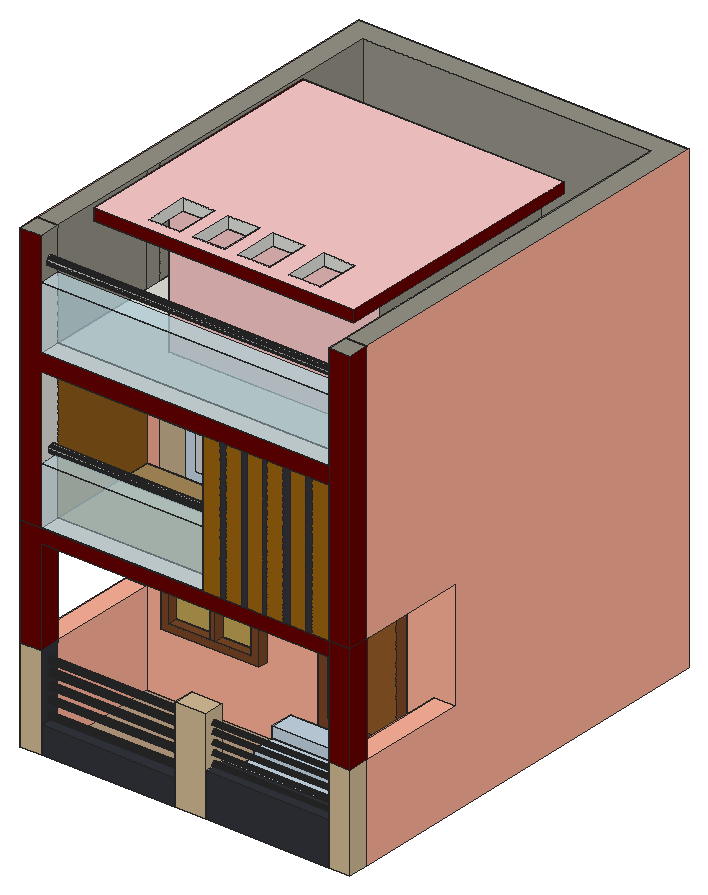
# SketchUp Ruby script. Lengths in inches.
U = 1.inch
M = Sketchup.active_model
def pt(a) = Geom::Point3d.new(a.map { |v| v * U })
def face(e, loops, mat)
  f = e.add_face(loops[0].map { |a| pt(a) })
  loops[1..].each { |l| e.add_face(l.map { |a| pt(a) }).erase! }
  f.material = f.back_material = mat if mat
  f
end
# faces: each face lists its corners as indices into pts; further lists are holes
def faces(e, pts, list, mat = nil) = list.each { |f| face(e, (f[0].is_a?(Array) ? f : [f]).map { |l| l.map { |i| pts[i] } }, mat) }
# xy, xz, yz: faces in a plane at the given z, y or x. An outline is a flat list of corners, or four numbers for a rectangle; further outlines are holes
def ring(l) = l.size == 4 ? [[l[0], l[1]], [l[2], l[1]], [l[2], l[3]], [l[0], l[3]]] : l.each_slice(2).to_a
def flat(e, list, mat, &to3) = list.each { |f| face(e, (f[0].is_a?(Array) ? f : [f]).map { |l| ring(l).map { |u, v| to3.(u, v) } }, mat) }
def xy(e, z, list, mat = nil) = flat(e, list, mat) { |x, y| [x, y, z] }
def xz(e, y, list, mat = nil) = flat(e, list, mat) { |x, z| [x, y, z] }
def yz(e, x, list, mat = nil) = flat(e, list, mat) { |y, z| [x, y, z] }
def lines(e, pts, list) = list.each { |a, b| e.add_line(pt(pts[a]), pt(pts[b])) }
# prism: a flat outline (further loops are holes) pulled along v
def prism(e, loops, v, mat = nil)
  f = face(e, loops, mat); d = Geom::Vector3d.new(v.map { |x| x * U })
  f.pushpull(f.normal.samedirection?(d) ? d.length : -d.length)
end
def box(e, o, s, mat = nil) = prism(e, [[o, [o[0] + s[0], o[1], o[2]], [o[0] + s[0], o[1] + s[1], o[2]], [o[0], o[1] + s[1], o[2]]]], [0, 0, s[2]], mat)
def at(x, y, z, deg = 0) = Geom::Transformation.translation(pt([x, y, z])) * Geom::Transformation.rotation(ORIGIN, Z_AXIS, deg.degrees)
def axes(o, x, y, z) = Geom::Transformation.new([*x, 0, *y, 0, *z, 0, *pt(o).to_a, 1])
def part(name) = M.definitions.add(name)
# library, detail: a bought-in or finely detailed component or shape, given as its bounding box
def library(name, o, s) = part(name).tap { |d| box(d.entities, o, s) }
def detail(e, o, s) = box(e.add_group.entities, o, s)
def put(e, d, t, mat = nil) = e.add_instance(d, t).tap { |i| i.material = mat if mat }
def group(e, t, mat = nil) = e.add_group.tap { |g| g.transformation = t; g.material = mat if mat }.entities
root = M.entities
M.materials.add("[Aluminum]").color = [179, 179, 179]
M.materials.add("[Blinds Cloth Horizontal]").color = [192, 163, 85]
M.materials.add("[Blinds Vertical Pattern]").color = [212, 212, 214]
M.materials.add("[Blinds Weave]").color = [141, 91, 25]
M.materials.add("[Blinds Wood Light]").color = [155, 100, 14]
M.materials.add("[Carpet Loop Pattern]").color = [166, 138, 89]
M.materials.add("[Carpet Pattern Leaf Squares Tan]").color = [181, 154, 125]
M.materials.add("[Color A01]").color = [255, 204, 204]
M.materials.add("[Color A08]").color = [102, 0, 0]
M.materials.add("[Color B02]").color = [255, 178, 153]
M.materials.add("[Color M08]").color = [30, 30, 30]
M.materials.add("[Formica Beige]").color = [211, 187, 149]
M.materials.add("[Formica Graystone]").color = [149, 146, 135]
M.materials.add("[Formica Laminate Dark]").color = [50, 53, 60]
M.materials.add("[Terrazzo Light Blue]").color = [196, 214, 227]
M.materials.add("[Translucent Glass Safety]").color = [204, 235, 244]
M.materials["[Translucent Glass Safety]"].alpha = 0.5
M.materials.add("[Wood Bamboo]").color = [177, 105, 43]
M.materials.add("[Wood Floor Light]").color = [204, 176, 127]
M.materials.add("[Wood Floor Parquet]").color = [145, 89, 39]
M.materials.add("[Wood Veneer 01]").color = [120, 70, 37]
xy(root,0,[[0,0,4.9375,4.9375],[4.9375,0,36.06,4.9375],[36.06,0,43.13,4.9375],[43.13,0,71.8125,4.9375],[71.8125,0,76.75,4.9375],
  [0,4.9375,4.9375,30.76],[71.8125,4.9375,76.75,30.76],[38.375,14.73,71.8125,20.02],[38.375,20.02,71.8125,25.31],[38.375,25.31,71.8125,30.76],
  [[0,30.76,76.75,98.62],[4.9375,34.47,71.8125,93.68]],[4.9375,34.47,71.8125,93.68]])
xy(root,0,[[4.9375,4.9375,71.8125,4.9375,71.8125,14.73,38.375,14.73,38.375,30.76,4.9375,30.76]],"[Carpet Pattern Leaf Squares Tan]")
xy(root,2.625,[[38.375,14.73,71.8125,20.02]],"[Terrazzo Light Blue]")
xy(root,4.125,[[38.375,20.02,71.8125,25.31]],"[Terrazzo Light Blue]")
xy(root,6.25,[[4.9375,0,36.06,4.9375]],"[Formica Laminate Dark]")
xy(root,6.61,[[44.6,30.76,65.48,34.47]])
xy(root,6.61,[[38.375,25.31,71.8125,30.76]],"[Terrazzo Light Blue]")
xy(root,10,[[43.13,0,71.8125,4.9375]],"[Formica Laminate Dark]")
xy(root,15.55,[[9.99,28.51,32.74,30.76]])
xy(root,17.3,[[21.37,28.51,22.64,30.76]])
xy(root,17.3,[[11.74,28.51,21.37,30.76],[22.64,28.51,31,30.76]],"[Wood Veneer 01]")
xy(root,21.74,[[0,0,4.9375,4.9375]])
xy(root,21.74,[[0,4.9375,4.9375,30.76]],"[Color B02]")
xy(root,21.97,[[71.8125,0,76.75,4.9375]])
xy(root,21.97,[[71.8125,4.9375,76.75,30.76]],"[Color B02]")
xy(root,21.97,[[36.06,0,43.13,4.9375]],"[Formica Beige]")
xy(root,37.87,[[11.74,28.51,21.37,30.76],[21.37,28.51,22.64,30.76],[22.64,28.51,31,30.76]])
xy(root,39.61,[[9.99,28.51,32.74,30.76]],"[Wood Veneer 01]")
xy(root,43.9375,[[4.9375,0,71.8125,4.9375],[4.9375,4.9375,71.8125,30.76]],"[Color A01]")
xy(root,44.67,[[44.6,30.76,65.48,34.47]])
xy(root,47.375,[[0,0,4.9375,4.9375],[4.9375,0,42.62,4.9375],[42.62,0,71.8125,4.9375],[71.8125,0,76.75,4.9375]])
xy(root,47.375,[[4.9375,4.9375,71.8125,30.76]],"[Carpet Loop Pattern]")
xy(root,47.375,[[0,4.9375,4.9375,30.76],[71.8125,4.9375,76.75,30.76]],"[Color A01]")
xy(root,60.75,[[4.9375,0,42.62,4.9375]],"[Translucent Glass Safety]")
xy(root,79.89,[[4.9375,0,42.62,4.9375]])
xy(root,83.8125,[[4.9375,0,71.8125,4.9375],[4.9375,4.9375,71.8125,4.9375,71.8125,15.02,22.6875,15.02,22.6875,61.77,71.8125,61.77,71.8125,93.68,4.9375,93.68],[22.6875,15.02,71.8125,61.77]])
xy(root,98.5625,[[4.9375,0,71.8125,4.9375]],"[Translucent Glass Safety]")
xy(root,108.3125,[[0,0,4.9375,4.9375],[71.8125,0,76.75,4.9375],[0,4.9375,4.9375,4.9375,4.9375,93.68,71.8125,93.68,71.8125,4.9375,76.75,4.9375,76.75,98.62,0,98.62]],"[Formica Graystone]")
xy(root,115.22,[[35.52,1.27,35.28,1.3,35.05,1.39,34.86,1.54,34.71,1.73,34.61,1.96,34.58,2.2,34.61,2.45,34.71,2.67,34.86,2.87,35.05,3.01,35.28,3.11,35.52,3.14,35.76,3.11,35.99,3.01,36.18,2.87,36.33,2.67,36.42,2.45,36.46,2.2,36.42,1.96,36.33,1.73,36.18,1.54,35.99,1.39,35.76,1.3],[45.96,1.27,45.71,1.3,45.49,1.39,45.29,1.54,45.14,1.73,45.05,1.96,45.02,2.2,45.05,2.45,45.14,2.67,45.29,2.87,45.49,3.01,45.71,3.11,45.96,3.14,46.2,3.11,46.43,3.01,46.62,2.87,46.77,2.67,46.86,2.45,46.89,2.2,46.86,1.96,46.77,1.73,46.62,1.54,46.43,1.39,46.2,1.3],[56.89,1.27,56.65,1.3,56.43,1.39,56.23,1.54,56.08,1.73,55.99,1.96,55.96,2.2,55.99,2.45,56.08,2.67,56.23,2.87,56.43,3.01,56.65,3.11,56.89,3.14,57.14,3.11,57.36,3.01,57.56,2.87,57.71,2.67,57.8,2.45,57.83,2.2,57.8,1.96,57.71,1.73,57.56,1.54,57.36,1.39,57.14,1.3],[72.48,2.38,72.24,2.41,72.01,2.5,71.82,2.65,71.67,2.85,71.57,3.07,71.54,3.32,71.57,3.56,71.67,3.78,71.82,3.98,72.01,4.13,72.24,4.22,72.48,4.25,72.72,4.22,72.95,4.13,73.14,3.98,73.29,3.78,73.38,3.56,73.42,3.32,73.38,3.07,73.29,2.85,73.14,2.65,72.95,2.5,72.72,2.41],[20.14,3.18,19.89,3.21,19.67,3.31,19.47,3.46,19.33,3.65,19.23,3.875,19.2,4.12,19.23,4.36,19.33,4.59,19.47,4.78,19.67,4.93,19.89,5.02,20.14,5.06,20.38,5.02,20.61,4.93,20.8,4.78,20.95,4.59,21.04,4.36,21.08,4.12,21.04,3.875,20.95,3.65,20.8,3.46,20.61,3.31,20.38,3.21]])
xy(root,115.22,[[[16.5,0.77,16.5,61.77,22.6875,61.77,22.6875,15.02,71.8125,15.02,71.8125,61.77,77.125,61.77,77.125,0.77],[26.97,3.62,34.28,13.74],[37.41,3.62,44.72,13.74],[47.91,3.62,55.22,13.74],[59.66,3.62,66.97,13.74],[20.14,3.18,20.38,3.21,20.61,3.31,20.8,3.46,20.95,3.65,21.04,3.875,21.08,4.12,21.04,4.36,20.95,4.59,20.8,4.78,20.61,4.93,20.38,5.02,20.14,5.06,19.89,5.02,19.67,4.93,19.47,4.78,19.33,4.59,19.23,4.36,19.2,4.12,19.23,3.875,19.33,3.65,19.47,3.46,19.67,3.31,19.89,3.21],[35.52,1.27,35.76,1.3,35.99,1.39,36.18,1.54,36.33,1.73,36.42,1.96,36.46,2.2,36.42,2.45,36.33,2.67,36.18,2.87,35.99,3.01,35.76,3.11,35.52,3.14,35.28,3.11,35.05,3.01,34.86,2.87,34.71,2.67,34.61,2.45,34.58,2.2,34.61,1.96,34.71,1.73,34.86,1.54,35.05,1.39,35.28,1.3],[45.96,1.27,46.2,1.3,46.43,1.39,46.62,1.54,46.77,1.73,46.86,1.96,46.89,2.2,46.86,2.45,46.77,2.67,46.62,2.87,46.43,3.01,46.2,3.11,45.96,3.14,45.71,3.11,45.49,3.01,45.29,2.87,45.14,2.67,45.05,2.45,45.02,2.2,45.05,1.96,45.14,1.73,45.29,1.54,45.49,1.39,45.71,1.3],[56.89,1.27,57.14,1.3,57.36,1.39,57.56,1.54,57.71,1.73,57.8,1.96,57.83,2.2,57.8,2.45,57.71,2.67,57.56,2.87,57.36,3.01,57.14,3.11,56.89,3.14,56.65,3.11,56.43,3.01,56.23,2.87,56.08,2.67,55.99,2.45,55.96,2.2,55.99,1.96,56.08,1.73,56.23,1.54,56.43,1.39,56.65,1.3],[72.48,2.38,72.72,2.41,72.95,2.5,73.14,2.65,73.29,2.85,73.38,3.07,73.42,3.32,73.38,3.56,73.29,3.78,73.14,3.98,72.95,4.13,72.72,4.22,72.48,4.25,72.24,4.22,72.01,4.13,71.82,3.98,71.67,3.78,71.57,3.56,71.54,3.32,71.57,3.07,71.67,2.85,71.82,2.65,72.01,2.5,72.24,2.41]]],"[Color A08]")
xy(root,117.875,[[[16.5,0.77,77.125,61.77],[26.97,3.62,34.28,13.74],[37.41,3.62,44.72,13.74],[47.91,3.62,55.22,13.74],[59.66,3.62,66.97,13.74]]],"[Color A01]")
xz(root,0,[[42.62,47.375,46.39,79.89],[47.81,47.375,51.58,79.89],[52.68,47.375,56.45,79.89],[57.49,47.375,61.27,79.89],[62.77,47.375,66.54,79.89],
  [68.04,47.375,71.8125,79.89]],"[Blinds Wood Light]")
xz(root,0,[[0,21.74,4.9375,21.74,4.9375,43.9375,71.8125,43.9375,71.8125,47.375,0,47.375],[71.8125,21.97,76.75,47.375],[0,47.375,4.9375,47.375,4.9375,79.89,71.8125,79.89,71.8125,83.8125,4.9375,83.8125,4.9375,108.3125,0,108.3125],[71.8125,47.375,76.75,108.3125]],"[Color A08]")
xz(root,0,[[0,0,4.9375,21.74],[36.06,0,43.13,21.97],[71.8125,0,76.75,21.97]],"[Formica Beige]")
xz(root,0,[[4.9375,0,36.06,6.25],[43.13,0,71.8125,10],[46.39,47.375,47.81,79.89],[51.58,47.375,52.68,79.89],[56.45,47.375,57.49,79.89],
  [61.27,47.375,62.77,79.89],[66.54,47.375,68.04,79.89]],"[Formica Laminate Dark]")
xz(root,0,[[4.9375,47.375,42.62,60.75],[4.9375,83.8125,71.8125,98.5625]],"[Translucent Glass Safety]")
xz(root,0.77,[[16.5,115.22,77.125,117.875]],"[Color A08]")
xz(root,3.62,[[26.97,115.22,34.28,117.875],[37.41,115.22,44.72,117.875],[47.91,115.22,55.22,117.875],[59.66,115.22,66.97,117.875]])
xz(root,4.9375,[[0,0,4.9375,21.74],[71.8125,0,76.75,21.97],[4.9375,43.9375,71.8125,47.375],[0,47.375,4.9375,83.8125],[42.62,47.375,71.8125,79.89],
  [71.8125,47.375,76.75,83.8125],[4.9375,79.89,71.8125,83.8125],[0,83.8125,4.9375,108.3125],[71.8125,83.8125,76.75,108.3125]])
xz(root,4.9375,[[0,21.74,4.9375,47.375],[71.8125,21.97,76.75,47.375]],"[Color A08]")
xz(root,4.9375,[[36.06,0,43.13,21.97]],"[Formica Beige]")
xz(root,4.9375,[[4.9375,0,36.06,6.25],[43.13,0,71.8125,10]],"[Formica Laminate Dark]")
xz(root,4.9375,[[4.9375,47.375,42.62,60.75],[4.9375,83.8125,71.8125,98.5625]],"[Translucent Glass Safety]")
xz(root,13.74,[[26.97,115.22,34.28,117.875],[37.41,115.22,44.72,117.875],[47.91,115.22,55.22,117.875],[59.66,115.22,66.97,117.875]])
xz(root,14.73,[[38.375,0,71.8125,2.625]],"[Terrazzo Light Blue]")
xz(root,15.02,[[22.6875,83.8125,71.8125,115.22]],"[Color A01]")
xz(root,20.02,[[38.375,0,71.8125,2.625]])
xz(root,20.02,[[38.375,2.625,71.8125,4.125]],"[Terrazzo Light Blue]")
xz(root,25.31,[[38.375,0,71.8125,4.125]])
xz(root,25.31,[[38.375,4.125,71.8125,6.61]],"[Terrazzo Light Blue]")
xz(root,28.51,[[[9.99,15.55,32.74,39.61],[11.74,17.3,31,37.87]],[21.37,17.3,22.64,37.87]],"[Wood Veneer 01]")
xz(root,30.76,[[0,0,4.9375,21.74],[38.375,0,71.8125,6.61],[[9.99,15.55,32.74,39.61],[11.74,17.3,31,37.87]],[21.37,17.3,22.64,37.87],[4.9375,43.9375,13.96,47.375],
  [13.96,43.9375,38.375,47.375],[38.375,43.9375,38.375,47.375,71.8125,47.375,71.8125,43.9375,65.48,43.9375,65.48,44.67,44.6,44.67,44.6,43.9375],[24.93,66.4,25.43,70.52],[26.99,66.4,27.49,70.52]])
xz(root,30.76,[[11.74,17.3,21.37,37.87],[22.64,17.3,31,37.87]],"[Blinds Cloth Horizontal]")
xz(root,30.76,[[16.02,49.43,24.11,78],[28.23,49.43,36.32,78]],"[Blinds Vertical Pattern]")
xz(root,30.76,[[[4.9375,0,38.375,0,38.375,6.61,44.6,6.61,44.6,43.9375,4.9375,43.9375,4.9375,47.375,0,47.375,0,21.74,4.9375,21.74],[9.99,15.55,32.74,39.61]],[65.48,6.61,71.8125,6.61,71.8125,21.97,76.75,21.97,76.75,47.375,71.8125,47.375,71.8125,43.9375,65.48,43.9375]],"[Color B02]")
xz(root,30.76,[[[13.96,47.375,26.17,80.06],[16.02,49.43,24.11,78],[24.93,66.4,25.43,70.52]],[[26.17,47.375,38.375,80.06],[28.23,49.43,36.32,78],[26.99,66.4,27.49,70.52]]],"[Terrazzo Light Blue]")
xz(root,30.76,[[48.54,21.62,49.85,31.37]],"[Wood Floor Light]")
xz(root,30.76,[[[47.12,9.13,62.96,42.15],[48.54,21.62,49.85,31.37]]],"[Wood Floor Parquet]")
xz(root,30.76,[[[44.6,6.61,65.48,43.9375],[47.12,9.13,62.96,42.15]],[44.6,43.9375,65.48,44.67]],"[Wood Veneer 01]")
xz(root,61.77,[[22.6875,83.8125,22.6875,115.22,16.5,115.22,16.5,117.875,77.125,117.875,77.125,115.22,71.8125,115.22,71.8125,83.8125]],"[Color A01]")
xz(root,93.68,[[4.9375,0,71.8125,83.8125]],"[Formica Beige]")
xz(root,93.68,[[4.9375,83.8125,71.8125,108.3125]],"[Formica Graystone]")
xz(root,98.62,[[0,0,76.75,108.3125]],"[Color B02]")
yz(root,0,[[0,21.74,4.9375,47.375],[0,47.375,4.9375,108.3125]],"[Color A08]")
yz(root,0,[[0,0,4.9375,21.74],[30.76,0,30.76,47.375,4.9375,47.375,4.9375,108.3125,98.62,108.3125,98.62,0],[4.9375,0,30.76,21.74]],"[Color B02]")
yz(root,4.9375,[[0,0,4.9375,6.25],[2.57,6.51,2.39,6.54,2.22,6.61,2.08,6.72,1.97,6.86,1.9,7.02,1.88,7.2,1.9,7.38,1.97,7.55,2.08,7.6875,2.22,7.8,2.39,7.87,2.57,7.89,2.74,7.87,2.91,7.8,3.05,7.6875,3.16,7.55,3.23,7.38,3.25,7.2,3.23,7.02,3.16,6.86,3.05,6.72,2.91,6.61,2.74,6.54],[2.57,9.83,2.39,9.85,2.22,9.92,2.08,10.03,1.97,10.17,1.9,10.34,1.88,10.51,1.9,10.69,1.97,10.86,2.08,11,2.22,11.11,2.39,11.18,2.57,11.2,2.74,11.18,2.91,11.11,3.05,11,3.16,10.86,3.23,10.69,3.25,10.51,3.23,10.34,3.16,10.17,3.05,10.03,2.91,9.92,2.74,9.85],[2.57,12.64,2.39,12.66,2.22,12.73,2.08,12.84,1.97,12.98,1.9,13.15,1.88,13.33,1.9,13.51,1.97,13.67,2.08,13.8125,2.22,13.92,2.39,13.99,2.57,14.01,2.74,13.99,2.91,13.92,3.05,13.8125,3.16,13.67,3.23,13.51,3.25,13.33,3.23,13.15,3.16,12.98,3.05,12.84,2.91,12.73,2.74,12.66],[2.57,15.51,2.39,15.54,2.22,15.61,2.08,15.72,1.97,15.86,1.9,16.02,1.88,16.2,1.9,16.38,1.97,16.55,2.08,16.6875,2.22,16.8,2.39,16.87,2.57,16.89,2.74,16.87,2.91,16.8,3.05,16.6875,3.16,16.55,3.23,16.38,3.25,16.2,3.23,16.02,3.16,15.86,3.05,15.72,2.91,15.61,2.74,15.54],
  [2.57,18.08,2.39,18.1,2.22,18.17,2.08,18.28,1.97,18.42,1.9,18.59,1.88,18.76,1.9,18.94,1.97,19.11,2.08,19.25,2.22,19.36,2.39,19.43,2.57,19.45,2.74,19.43,2.91,19.36,3.05,19.25,3.16,19.11,3.23,18.94,3.25,18.76,3.23,18.59,3.16,18.42,3.05,18.28,2.91,18.17,2.74,18.1],[4.9375,43.9375,30.76,47.375],[0,47.375,4.9375,60.75],[[0,60.75,4.9375,79.89],[2.8,61.9,2.56,61.93,2.33,62.02,2.14,62.17,1.99,62.37,1.9,62.59,1.86,62.84,1.9,63.08,1.99,63.3,2.14,63.5,2.33,63.65,2.56,63.74,2.8,63.77,3.04,63.74,3.27,63.65,3.46,63.5,3.61,63.3,3.71,63.08,3.74,62.84,3.71,62.59,3.61,62.37,3.46,62.17,3.27,62.02,3.04,61.93]],[0,83.8125,4.9375,98.5625],
  [2.36,101.3,2.12,101.34,1.89,101.43,1.7,101.58,1.55,101.77,1.45,102,1.42,102.24,1.45,102.48,1.55,102.71,1.7,102.9,1.89,103.05,2.12,103.15,2.36,103.18,2.6,103.15,2.83,103.05,3.02,102.9,3.17,102.71,3.26,102.48,3.3,102.24,3.26,102,3.17,101.77,3.02,101.58,2.83,101.43,2.6,101.34]])
yz(root,4.9375,[[4.9375,47.375,30.76,83.8125]],"[Blinds Weave]")
yz(root,4.9375,[[0,21.74,4.9375,43.9375]],"[Color A08]")
yz(root,4.9375,[[4.9375,0,30.76,21.74]],"[Color B02]")
yz(root,4.9375,[[34.47,0,93.68,83.8125]],"[Formica Beige]")
yz(root,4.9375,[[4.9375,83.8125,30.76,108.3125],[30.76,83.8125,34.47,108.3125],[34.47,83.8125,93.68,108.3125],[[0,98.5625,4.9375,108.3125],[2.36,101.3,2.12,101.34,1.89,101.43,1.7,101.58,1.55,101.77,1.45,102,1.42,102.24,1.45,102.48,1.55,102.71,1.7,102.9,1.89,103.05,2.12,103.15,2.36,103.18,2.6,103.15,2.83,103.05,3.02,102.9,3.17,102.71,3.26,102.48,3.3,102.24,3.26,102,3.17,101.77,3.02,101.58,2.83,101.43,2.6,101.34]]],"[Formica Graystone]")
yz(root,4.9375,[[[0,6.25,4.9375,21.74],[2.57,18.08,2.39,18.1,2.22,18.17,2.08,18.28,1.97,18.42,1.9,18.59,1.88,18.76,1.9,18.94,1.97,19.11,2.08,19.25,2.22,19.36,2.39,19.43,2.57,19.45,2.74,19.43,2.91,19.36,3.05,19.25,3.16,19.11,3.23,18.94,3.25,18.76,3.23,18.59,3.16,18.42,3.05,18.28,2.91,18.17,2.74,18.1],[2.57,15.51,2.39,15.54,2.22,15.61,2.08,15.72,1.97,15.86,1.9,16.02,1.88,16.2,1.9,16.38,1.97,16.55,2.08,16.6875,2.22,16.8,2.39,16.87,2.57,16.89,2.74,16.87,2.91,16.8,3.05,16.6875,3.16,16.55,3.23,16.38,3.25,16.2,3.23,16.02,3.16,15.86,3.05,15.72,2.91,15.61,2.74,15.54],[2.57,12.64,2.39,12.66,2.22,12.73,2.08,12.84,1.97,12.98,1.9,13.15,1.88,13.33,1.9,13.51,1.97,13.67,2.08,13.8125,2.22,13.92,2.39,13.99,2.57,14.01,2.74,13.99,2.91,13.92,3.05,13.8125,3.16,13.67,3.23,13.51,3.25,13.33,3.23,13.15,3.16,12.98,3.05,12.84,2.91,12.73,2.74,12.66],[2.57,9.83,2.39,9.85,2.22,9.92,2.08,10.03,1.97,10.17,1.9,10.34,1.88,10.51,1.9,10.69,1.97,10.86,2.08,11,2.22,11.11,2.39,11.18,2.57,11.2,2.74,11.18,2.91,11.11,3.05,11,3.16,10.86,3.23,10.69,3.25,10.51,3.23,10.34,3.16,10.17,3.05,10.03,2.91,9.92,2.74,9.85],[2.57,6.51,2.39,6.54,2.22,6.61,2.08,6.72,1.97,6.86,1.9,7.02,1.88,7.2,1.9,7.38,1.97,7.55,2.08,7.6875,2.22,7.8,2.39,7.87,2.57,7.89,2.74,7.87,2.91,7.8,3.05,7.6875,3.16,7.55,3.23,7.38,3.25,7.2,3.23,7.02,3.16,6.86,3.05,6.72,2.91,6.61,2.74,6.54]]],"[Formica Laminate Dark]")
yz(root,9.99,[[28.51,15.55,30.76,39.61]],"[Wood Veneer 01]")
yz(root,11.74,[[28.51,17.3,30.76,37.87]],"[Wood Veneer 01]")
yz(root,16.5,[[0.77,115.22,61.77,117.875]],"[Color A08]")
yz(root,21.37,[[28.51,17.3,30.76,37.87]],"[Wood Veneer 01]")
yz(root,22.64,[[28.51,17.3,30.76,37.87]],"[Wood Veneer 01]")
yz(root,22.6875,[[15.02,83.8125,61.77,115.22]],"[Color A01]")
yz(root,26.97,[[3.62,115.22,13.74,117.875]])
yz(root,31,[[28.51,17.3,30.76,37.87]],"[Wood Veneer 01]")
yz(root,32.74,[[28.51,15.55,30.76,39.61]],"[Wood Veneer 01]")
yz(root,34.28,[[3.62,115.22,13.74,117.875]])
yz(root,36.06,[[0,0,4.9375,6.25]])
yz(root,36.06,[[[0,6.25,4.9375,21.97],[2.57,18.08,2.74,18.1,2.91,18.17,3.05,18.28,3.16,18.42,3.23,18.59,3.25,18.76,3.23,18.94,3.16,19.11,3.05,19.25,2.91,19.36,2.74,19.43,2.57,19.45,2.39,19.43,2.22,19.36,2.08,19.25,1.97,19.11,1.9,18.94,1.88,18.76,1.9,18.59,1.97,18.42,2.08,18.28,2.22,18.17,2.39,18.1],[2.57,15.51,2.74,15.54,2.91,15.61,3.05,15.72,3.16,15.86,3.23,16.02,3.25,16.2,3.23,16.38,3.16,16.55,3.05,16.6875,2.91,16.8,2.74,16.87,2.57,16.89,2.39,16.87,2.22,16.8,2.08,16.6875,1.97,16.55,1.9,16.38,1.88,16.2,1.9,16.02,1.97,15.86,2.08,15.72,2.22,15.61,2.39,15.54],[2.57,12.64,2.74,12.66,2.91,12.73,3.05,12.84,3.16,12.98,3.23,13.15,3.25,13.33,3.23,13.51,3.16,13.67,3.05,13.8125,2.91,13.92,2.74,13.99,2.57,14.01,2.39,13.99,2.22,13.92,2.08,13.8125,1.97,13.67,1.9,13.51,1.88,13.33,1.9,13.15,1.97,12.98,2.08,12.84,2.22,12.73,2.39,12.66],[2.57,9.83,2.74,9.85,2.91,9.92,3.05,10.03,3.16,10.17,3.23,10.34,3.25,10.51,3.23,10.69,3.16,10.86,3.05,11,2.91,11.11,2.74,11.18,2.57,11.2,2.39,11.18,2.22,11.11,2.08,11,1.97,10.86,1.9,10.69,1.88,10.51,1.9,10.34,1.97,10.17,2.08,10.03,2.22,9.92,2.39,9.85],[2.57,6.51,2.74,6.54,2.91,6.61,3.05,6.72,3.16,6.86,3.23,7.02,3.25,7.2,3.23,7.38,3.16,7.55,3.05,7.6875,2.91,7.8,2.74,7.87,2.57,7.89,2.39,7.87,2.22,7.8,2.08,7.6875,1.97,7.55,1.9,7.38,1.88,7.2,1.9,7.02,1.97,6.86,2.08,6.72,2.22,6.61,2.39,6.54]]],"[Formica Beige]")
yz(root,37.41,[[3.62,115.22,13.74,117.875]])
yz(root,38.375,[[14.73,0,20.02,2.625],[20.02,0,25.31,4.125],[25.31,0,30.76,6.61]],"[Terrazzo Light Blue]")
yz(root,42.62,[[0,47.375,4.9375,60.75]])
yz(root,42.62,[[[0,60.75,4.9375,79.89],[2.8,61.9,3.04,61.93,3.27,62.02,3.46,62.17,3.61,62.37,3.71,62.59,3.74,62.84,3.71,63.08,3.61,63.3,3.46,63.5,3.27,63.65,3.04,63.74,2.8,63.77,2.56,63.74,2.33,63.65,2.14,63.5,1.99,63.3,1.9,63.08,1.86,62.84,1.9,62.59,1.99,62.37,2.14,62.17,2.33,62.02,2.56,61.93]],[2.8,61.9,3.04,61.93,3.27,62.02,3.46,62.17,3.61,62.37,3.71,62.59,3.74,62.84,3.71,63.08,3.61,63.3,3.46,63.5,3.27,63.65,3.04,63.74,2.8,63.77,2.56,63.74,2.33,63.65,2.14,63.5,1.99,63.3,1.9,63.08,1.86,62.84,1.9,62.59,1.99,62.37,2.14,62.17,2.33,62.02,2.56,61.93]],"[Wood Bamboo]")
yz(root,43.13,[[0,0,4.9375,10],[2.32,10.2,2.21,10.21,2.1,10.26,2.01,10.33,1.94,10.42,1.9,10.52,1.88,10.64,1.9,10.75,1.94,10.86,2.01,10.95,2.1,11.02,2.21,11.06,2.32,11.07,2.43,11.06,2.54,11.02,2.63,10.95,2.7,10.86,2.74,10.75,2.76,10.64,2.74,10.52,2.7,10.42,2.63,10.33,2.54,10.26,2.43,10.21],[2.32,12.45,2.21,12.46,2.1,12.51,2.01,12.58,1.94,12.67,1.9,12.77,1.88,12.89,1.9,13,1.94,13.11,2.01,13.2,2.1,13.27,2.21,13.31,2.32,13.32,2.43,13.31,2.54,13.27,2.63,13.2,2.7,13.11,2.74,13,2.76,12.89,2.74,12.77,2.7,12.67,2.63,12.58,2.54,12.51,2.43,12.46],[2.32,14.64,2.21,14.65,2.1,14.7,2.01,14.77,1.94,14.86,1.9,14.96,1.88,15.07,1.9,15.1875,1.94,15.29,2.01,15.38,2.1,15.45,2.21,15.5,2.32,15.51,2.43,15.5,2.54,15.45,2.63,15.38,2.7,15.29,2.74,15.1875,2.76,15.07,2.74,14.96,2.7,14.86,2.63,14.77,2.54,14.7,2.43,14.65],[2.32,16.89,2.21,16.9,2.1,16.95,2.01,17.02,1.94,17.11,1.9,17.21,1.88,17.32,1.9,17.4375,1.94,17.54,2.01,17.63,2.1,17.7,2.21,17.75,2.32,17.76,2.43,17.75,2.54,17.7,2.63,17.63,2.7,17.54,2.74,17.4375,2.76,17.32,2.74,17.21,2.7,17.11,2.63,17.02,2.54,16.95,2.43,16.9],
  [2.32,18.76,2.21,18.78,2.1,18.82,2.01,18.89,1.94,18.98,1.9,19.09,1.88,19.2,1.9,19.3125,1.94,19.42,2.01,19.51,2.1,19.58,2.21,19.62,2.32,19.64,2.43,19.62,2.54,19.58,2.63,19.51,2.7,19.42,2.74,19.3125,2.76,19.2,2.74,19.09,2.7,18.98,2.63,18.89,2.54,18.82,2.43,18.78]])
yz(root,43.13,[[[0,10,4.9375,21.97],[2.32,16.89,2.21,16.9,2.1,16.95,2.01,17.02,1.94,17.11,1.9,17.21,1.88,17.32,1.9,17.4375,1.94,17.54,2.01,17.63,2.1,17.7,2.21,17.75,2.32,17.76,2.43,17.75,2.54,17.7,2.63,17.63,2.7,17.54,2.74,17.4375,2.76,17.32,2.74,17.21,2.7,17.11,2.63,17.02,2.54,16.95,2.43,16.9],[2.32,14.64,2.21,14.65,2.1,14.7,2.01,14.77,1.94,14.86,1.9,14.96,1.88,15.07,1.9,15.1875,1.94,15.29,2.01,15.38,2.1,15.45,2.21,15.5,2.32,15.51,2.43,15.5,2.54,15.45,2.63,15.38,2.7,15.29,2.74,15.1875,2.76,15.07,2.74,14.96,2.7,14.86,2.63,14.77,2.54,14.7,2.43,14.65],[2.32,12.45,2.21,12.46,2.1,12.51,2.01,12.58,1.94,12.67,1.9,12.77,1.88,12.89,1.9,13,1.94,13.11,2.01,13.2,2.1,13.27,2.21,13.31,2.32,13.32,2.43,13.31,2.54,13.27,2.63,13.2,2.7,13.11,2.74,13,2.76,12.89,2.74,12.77,2.7,12.67,2.63,12.58,2.54,12.51,2.43,12.46],[2.32,10.2,2.21,10.21,2.1,10.26,2.01,10.33,1.94,10.42,1.9,10.52,1.88,10.64,1.9,10.75,1.94,10.86,2.01,10.95,2.1,11.02,2.21,11.06,2.32,11.07,2.43,11.06,2.54,11.02,2.63,10.95,2.7,10.86,2.74,10.75,2.76,10.64,2.74,10.52,2.7,10.42,2.63,10.33,2.54,10.26,2.43,10.21],[2.32,18.76,2.21,18.78,2.1,18.82,2.01,18.89,1.94,18.98,1.9,19.09,1.88,19.2,1.9,19.3125,1.94,19.42,2.01,19.51,2.1,19.58,2.21,19.62,2.32,19.64,2.43,19.62,2.54,19.58,2.63,19.51,2.7,19.42,2.74,19.3125,2.76,19.2,2.74,19.09,2.7,18.98,2.63,18.89,2.54,18.82,2.43,18.78]]],"[Formica Beige]")
yz(root,44.6,[[30.76,6.61,34.47,44.67]])
yz(root,44.72,[[3.62,115.22,13.74,117.875]])
yz(root,47.91,[[3.62,115.22,13.74,117.875]])
yz(root,55.22,[[3.62,115.22,13.74,117.875]])
yz(root,59.66,[[3.62,115.22,13.74,117.875]])
yz(root,65.48,[[30.76,6.61,34.47,44.67]])
yz(root,66.97,[[3.62,115.22,13.74,117.875]])
yz(root,71.8125,[[0,0,4.9375,10],[34.47,0,93.68,83.8125],[0,47.375,4.9375,79.89],[4.9375,47.375,30.76,83.8125],[0,83.8125,4.9375,98.5625],
  [15.02,83.8125,30.76,108.3125],[30.76,83.8125,34.47,108.3125],[34.47,83.8125,61.77,108.3125]])
yz(root,71.8125,[[4.9375,43.9375,30.76,47.375]],"[Color A01]")
yz(root,71.8125,[[0,21.97,4.9375,43.9375]],"[Color A08]")
yz(root,71.8125,[[4.9375,0,14.73,21.97],[14.73,2.625,20.02,21.97],[20.02,4.125,25.31,21.97],[25.31,6.61,30.76,21.97]],"[Color B02]")
yz(root,71.8125,[[[0,10,4.9375,21.97],[2.32,10.2,2.43,10.21,2.54,10.26,2.63,10.33,2.7,10.42,2.74,10.52,2.76,10.64,2.74,10.75,2.7,10.86,2.63,10.95,2.54,11.02,2.43,11.06,2.32,11.07,2.21,11.06,2.1,11.02,2.01,10.95,1.94,10.86,1.9,10.75,1.88,10.64,1.9,10.52,1.94,10.42,2.01,10.33,2.1,10.26,2.21,10.21],[2.32,18.76,2.43,18.78,2.54,18.82,2.63,18.89,2.7,18.98,2.74,19.09,2.76,19.2,2.74,19.3125,2.7,19.42,2.63,19.51,2.54,19.58,2.43,19.62,2.32,19.64,2.21,19.62,2.1,19.58,2.01,19.51,1.94,19.42,1.9,19.3125,1.88,19.2,1.9,19.09,1.94,18.98,2.01,18.89,2.1,18.82,2.21,18.78],[2.32,16.89,2.43,16.9,2.54,16.95,2.63,17.02,2.7,17.11,2.74,17.21,2.76,17.32,2.74,17.4375,2.7,17.54,2.63,17.63,2.54,17.7,2.43,17.75,2.32,17.76,2.21,17.75,2.1,17.7,2.01,17.63,1.94,17.54,1.9,17.4375,1.88,17.32,1.9,17.21,1.94,17.11,2.01,17.02,2.1,16.95,2.21,16.9],[2.32,14.64,2.43,14.65,2.54,14.7,2.63,14.77,2.7,14.86,2.74,14.96,2.76,15.07,2.74,15.1875,2.7,15.29,2.63,15.38,2.54,15.45,2.43,15.5,2.32,15.51,2.21,15.5,2.1,15.45,2.01,15.38,1.94,15.29,1.9,15.1875,1.88,15.07,1.9,14.96,1.94,14.86,2.01,14.77,2.1,14.7,2.21,14.65],[2.32,12.45,2.43,12.46,2.54,12.51,2.63,12.58,2.7,12.67,2.74,12.77,2.76,12.89,2.74,13,2.7,13.11,2.63,13.2,2.54,13.27,2.43,13.31,2.32,13.32,2.21,13.31,2.1,13.27,2.01,13.2,1.94,13.11,1.9,13,1.88,12.89,1.9,12.77,1.94,12.67,2.01,12.58,2.1,12.51,2.21,12.46]]],"[Formica Beige]")
yz(root,71.8125,[[4.9375,83.8125,15.02,108.3125],[61.77,83.8125,93.68,108.3125],[[0,98.5625,4.9375,108.3125],[2.36,101.3,2.6,101.34,2.83,101.43,3.02,101.58,3.17,101.77,3.26,102,3.3,102.24,3.26,102.48,3.17,102.71,3.02,102.9,2.83,103.05,2.6,103.15,2.36,103.18,2.12,103.15,1.89,103.05,1.7,102.9,1.55,102.71,1.45,102.48,1.42,102.24,1.45,102,1.55,101.77,1.7,101.58,1.89,101.43,2.12,101.34]],[15.02,108.3125,61.77,115.22]],"[Formica Graystone]")
yz(root,71.8125,[[14.73,0,20.02,2.625],[20.02,0,25.31,4.125],[25.31,0,30.76,6.61]],"[Terrazzo Light Blue]")
yz(root,76.75,[[0,21.97,4.9375,47.375],[0,47.375,4.9375,108.3125]],"[Color A08]")
yz(root,76.75,[[4.9375,0,98.62,0,98.62,108.3125,4.9375,108.3125,4.9375,47.375,30.76,47.375,30.76,21.97,4.9375,21.97]],"[Color B02]")
yz(root,76.75,[[0,0,4.9375,21.97]],"[Formica Beige]")
yz(root,77.125,[[0.77,115.22,61.77,117.875]],"[Color A08]")
p = [[4.9375,2.22,6.61],[4.9375,2.39,6.54],[36.06,2.39,6.54],[36.06,2.22,6.61],[4.9375,2.57,6.51],[36.06,2.57,6.51],
  [4.9375,2.74,6.54],[36.06,2.74,6.54],[4.9375,2.91,6.61],[36.06,2.91,6.61],[4.9375,2.08,6.72],[36.06,2.08,6.72],
  [4.9375,3.05,6.72],[36.06,3.05,6.72],[4.9375,1.97,6.86],[36.06,1.97,6.86],[4.9375,3.16,6.86],[36.06,3.16,6.86],
  [4.9375,1.9,7.02],[36.06,1.9,7.02],[4.9375,3.23,7.02],[36.06,3.23,7.02],[4.9375,1.88,7.2],[36.06,1.88,7.2],
  [4.9375,3.25,7.2],[36.06,3.25,7.2],[4.9375,1.9,7.38],[36.06,1.9,7.38],[4.9375,3.23,7.38],[36.06,3.23,7.38],
  [4.9375,1.97,7.55],[36.06,1.97,7.55],[4.9375,3.16,7.55],[36.06,3.16,7.55],[4.9375,2.08,7.6875],[36.06,2.08,7.6875],
  [4.9375,3.05,7.6875],[36.06,3.05,7.6875],[4.9375,2.22,7.8],[36.06,2.22,7.8],[4.9375,2.91,7.8],[36.06,2.91,7.8],
  [4.9375,2.39,7.87],[36.06,2.39,7.87],[4.9375,2.74,7.87],[36.06,2.74,7.87],[4.9375,2.57,7.89],[36.06,2.57,7.89],
  [4.9375,2.39,9.85],[4.9375,2.57,9.83],[36.06,2.57,9.83],[36.06,2.39,9.85],[4.9375,2.74,9.85],[36.06,2.74,9.85],
  [4.9375,2.08,10.03],[4.9375,2.22,9.92],[36.06,2.22,9.92],[36.06,2.08,10.03],[4.9375,2.91,9.92],[36.06,2.91,9.92],
  [4.9375,3.05,10.03],[36.06,3.05,10.03],[4.9375,1.97,10.17],[36.06,1.97,10.17],[4.9375,3.16,10.17],[36.06,3.16,10.17],
  [4.9375,1.9,10.34],[36.06,1.9,10.34],[43.13,2.1,10.26],[43.13,2.21,10.21],[71.8125,2.21,10.21],[71.8125,2.1,10.26],
  [43.13,2.32,10.2],[71.8125,2.32,10.2],[43.13,2.43,10.21],[71.8125,2.43,10.21],[43.13,2.54,10.26],[71.8125,2.54,10.26],
  [4.9375,3.23,10.34],[36.06,3.23,10.34],[4.9375,1.88,10.51],[36.06,1.88,10.51],[43.13,1.94,10.42],[43.13,2.01,10.33],
  [71.8125,2.01,10.33],[71.8125,1.94,10.42],[43.13,2.63,10.33],[71.8125,2.63,10.33],[43.13,2.7,10.42],[71.8125,2.7,10.42],
  [4.9375,3.25,10.51],[36.06,3.25,10.51],[43.13,1.9,10.52],[71.8125,1.9,10.52],[43.13,2.74,10.52],[71.8125,2.74,10.52],
  [4.9375,1.9,10.69],[36.06,1.9,10.69],[43.13,1.88,10.64],[71.8125,1.88,10.64],[43.13,2.76,10.64],[71.8125,2.76,10.64],
  [4.9375,3.23,10.69],[36.06,3.23,10.69],[43.13,1.9,10.75],[71.8125,1.9,10.75],[43.13,2.74,10.75],[71.8125,2.74,10.75],
  [4.9375,1.97,10.86],[36.06,1.97,10.86],[4.9375,3.16,10.86],[36.06,3.16,10.86],[43.13,1.94,10.86],[71.8125,1.94,10.86],
  [43.13,2.7,10.86],[71.8125,2.7,10.86],[43.13,2.01,10.95],[71.8125,2.01,10.95],[4.9375,2.08,11],[36.06,2.08,11],
  [43.13,2.1,11.02],[71.8125,2.1,11.02],[43.13,2.63,10.95],[43.13,2.54,11.02],[71.8125,2.54,11.02],[71.8125,2.63,10.95],
  [4.9375,3.05,11],[36.06,3.05,11],[4.9375,2.22,11.11],[36.06,2.22,11.11],[43.13,2.21,11.06],[71.8125,2.21,11.06],
  [43.13,2.43,11.06],[71.8125,2.43,11.06],[4.9375,2.91,11.11],[36.06,2.91,11.11],[4.9375,2.39,11.18],[36.06,2.39,11.18],
  [43.13,2.32,11.07],[71.8125,2.32,11.07],[4.9375,2.74,11.18],[36.06,2.74,11.18],[4.9375,2.57,11.2],[36.06,2.57,11.2],
  [43.13,2.21,12.46],[43.13,2.32,12.45],[71.8125,2.32,12.45],[71.8125,2.21,12.46],[43.13,2.43,12.46],[71.8125,2.43,12.46],
  [43.13,2.01,12.58],[43.13,2.1,12.51],[71.8125,2.1,12.51],[71.8125,2.01,12.58],[43.13,2.54,12.51],[71.8125,2.54,12.51],
  [43.13,2.63,12.58],[71.8125,2.63,12.58],[43.13,1.94,12.67],[71.8125,1.94,12.67],[4.9375,2.39,12.66],[4.9375,2.57,12.64],
  [36.06,2.57,12.64],[36.06,2.39,12.66],[4.9375,2.74,12.66],[36.06,2.74,12.66],[43.13,2.7,12.67],[71.8125,2.7,12.67],
  [43.13,1.9,12.77],[71.8125,1.9,12.77],[4.9375,2.08,12.84],[4.9375,2.22,12.73],[36.06,2.22,12.73],[36.06,2.08,12.84],
  [4.9375,2.91,12.73],[36.06,2.91,12.73],[43.13,2.74,12.77],[71.8125,2.74,12.77],[4.9375,3.05,12.84],[36.06,3.05,12.84],
  [43.13,1.88,12.89],[71.8125,1.88,12.89],[4.9375,1.97,12.98],[36.06,1.97,12.98],[43.13,2.76,12.89],[71.8125,2.76,12.89],
  [4.9375,3.16,12.98],[36.06,3.16,12.98],[43.13,1.9,13],[71.8125,1.9,13],[43.13,2.74,13],[71.8125,2.74,13],
  [4.9375,1.9,13.15],[36.06,1.9,13.15],[43.13,1.94,13.11],[71.8125,1.94,13.11],[43.13,2.7,13.11],[71.8125,2.7,13.11],
  [4.9375,3.23,13.15],[36.06,3.23,13.15],[4.9375,1.88,13.33],[36.06,1.88,13.33],[43.13,2.01,13.2],[71.8125,2.01,13.2],
  [43.13,2.63,13.2],[71.8125,2.63,13.2],[4.9375,3.25,13.33],[36.06,3.25,13.33],[43.13,2.1,13.27],[71.8125,2.1,13.27],
  [43.13,2.54,13.27],[71.8125,2.54,13.27],[4.9375,1.9,13.51],[36.06,1.9,13.51],[43.13,2.21,13.31],[71.8125,2.21,13.31],
  [43.13,2.32,13.32],[71.8125,2.32,13.32],[43.13,2.43,13.31],[71.8125,2.43,13.31],[4.9375,3.23,13.51],[36.06,3.23,13.51],
  [4.9375,1.97,13.67],[36.06,1.97,13.67],[4.9375,3.16,13.67],[36.06,3.16,13.67],[4.9375,2.08,13.8125],[36.06,2.08,13.8125],
  [4.9375,3.05,13.8125],[36.06,3.05,13.8125],[4.9375,2.22,13.92],[36.06,2.22,13.92],[4.9375,2.91,13.92],[36.06,2.91,13.92],
  [4.9375,2.39,13.99],[36.06,2.39,13.99],[4.9375,2.74,13.99],[36.06,2.74,13.99],[4.9375,2.57,14.01],[36.06,2.57,14.01],
  [43.13,2.21,14.65],[43.13,2.32,14.64],[71.8125,2.32,14.64],[71.8125,2.21,14.65],[43.13,2.43,14.65],[71.8125,2.43,14.65],
  [43.13,2.01,14.77],[43.13,2.1,14.7],[71.8125,2.1,14.7],[71.8125,2.01,14.77],[43.13,2.54,14.7],[71.8125,2.54,14.7],
  [43.13,2.63,14.77],[71.8125,2.63,14.77],[43.13,1.94,14.86],[71.8125,1.94,14.86],[43.13,2.7,14.86],[71.8125,2.7,14.86],
  [43.13,1.9,14.96],[71.8125,1.9,14.96],[43.13,2.74,14.96],[71.8125,2.74,14.96],[43.13,1.88,15.07],[71.8125,1.88,15.07],
  [43.13,2.76,15.07],[71.8125,2.76,15.07],[43.13,1.9,15.1875],[71.8125,1.9,15.1875],[43.13,2.74,15.1875],[71.8125,2.74,15.1875],
  [43.13,1.94,15.29],[71.8125,1.94,15.29],[43.13,2.7,15.29],[71.8125,2.7,15.29],[43.13,2.01,15.38],[71.8125,2.01,15.38],
  [43.13,2.63,15.38],[71.8125,2.63,15.38],[43.13,2.1,15.45],[71.8125,2.1,15.45],[43.13,2.54,15.45],[71.8125,2.54,15.45],
  [43.13,2.21,15.5],[71.8125,2.21,15.5],[4.9375,2.22,15.61],[4.9375,2.39,15.54],[36.06,2.39,15.54],[36.06,2.22,15.61],
  [43.13,2.32,15.51],[71.8125,2.32,15.51],[43.13,2.43,15.5],[71.8125,2.43,15.5],[4.9375,2.57,15.51],[36.06,2.57,15.51],
  [4.9375,2.74,15.54],[36.06,2.74,15.54],[4.9375,2.91,15.61],[36.06,2.91,15.61],[4.9375,2.08,15.72],[36.06,2.08,15.72],
  [4.9375,3.05,15.72],[36.06,3.05,15.72],[4.9375,1.97,15.86],[36.06,1.97,15.86],[4.9375,3.16,15.86],[36.06,3.16,15.86],
  [4.9375,1.9,16.02],[36.06,1.9,16.02],[4.9375,3.23,16.02],[36.06,3.23,16.02],[4.9375,1.88,16.2],[36.06,1.88,16.2],
  [4.9375,3.25,16.2],[36.06,3.25,16.2],[4.9375,1.9,16.38],[36.06,1.9,16.38],[4.9375,3.23,16.38],[36.06,3.23,16.38],
  [4.9375,1.97,16.55],[36.06,1.97,16.55],[4.9375,3.16,16.55],[36.06,3.16,16.55],[4.9375,2.08,16.6875],[36.06,2.08,16.6875],
  [4.9375,3.05,16.6875],[36.06,3.05,16.6875],[4.9375,2.22,16.8],[36.06,2.22,16.8],[4.9375,2.91,16.8],[36.06,2.91,16.8],
  [4.9375,2.39,16.87],[36.06,2.39,16.87],[4.9375,2.74,16.87],[36.06,2.74,16.87],[43.13,2.01,17.02],[43.13,2.1,16.95],
  [71.8125,2.1,16.95],[71.8125,2.01,17.02],[43.13,2.21,16.9],[71.8125,2.21,16.9],[43.13,2.32,16.89],[71.8125,2.32,16.89],
  [43.13,2.43,16.9],[71.8125,2.43,16.9],[4.9375,2.57,16.89],[36.06,2.57,16.89],[43.13,2.54,16.95],[71.8125,2.54,16.95],
  [43.13,2.63,17.02],[71.8125,2.63,17.02],[43.13,1.94,17.11],[71.8125,1.94,17.11],[43.13,2.7,17.11],[71.8125,2.7,17.11],
  [43.13,1.9,17.21],[71.8125,1.9,17.21],[43.13,2.74,17.21],[71.8125,2.74,17.21],[43.13,1.88,17.32],[71.8125,1.88,17.32],
  [43.13,2.76,17.32],[71.8125,2.76,17.32],[43.13,1.9,17.4375],[71.8125,1.9,17.4375],[43.13,2.74,17.4375],[71.8125,2.74,17.4375],
  [43.13,1.94,17.54],[71.8125,1.94,17.54],[43.13,2.7,17.54],[71.8125,2.7,17.54],[43.13,2.01,17.63],[71.8125,2.01,17.63],
  [43.13,2.63,17.63],[71.8125,2.63,17.63],[43.13,2.1,17.7],[71.8125,2.1,17.7],[43.13,2.54,17.7],[71.8125,2.54,17.7],
  [43.13,2.21,17.75],[71.8125,2.21,17.75],[43.13,2.32,17.76],[71.8125,2.32,17.76],[43.13,2.43,17.75],[71.8125,2.43,17.75],
  [4.9375,2.22,18.17],[4.9375,2.39,18.1],[36.06,2.39,18.1],[36.06,2.22,18.17],[4.9375,2.57,18.08],[36.06,2.57,18.08],
  [4.9375,2.74,18.1],[36.06,2.74,18.1],[4.9375,2.91,18.17],[36.06,2.91,18.17],[4.9375,2.08,18.28],[36.06,2.08,18.28],
  [4.9375,3.05,18.28],[36.06,3.05,18.28],[4.9375,1.97,18.42],[36.06,1.97,18.42],[4.9375,3.16,18.42],[36.06,3.16,18.42],
  [4.9375,1.9,18.59],[36.06,1.9,18.59],[4.9375,3.23,18.59],[36.06,3.23,18.59],[4.9375,1.88,18.76],[36.06,1.88,18.76],
  [4.9375,3.25,18.76],[36.06,3.25,18.76],[4.9375,1.9,18.94],[36.06,1.9,18.94],[43.13,2.01,18.89],[43.13,2.1,18.82],
  [71.8125,2.1,18.82],[71.8125,2.01,18.89],[43.13,2.21,18.78],[71.8125,2.21,18.78],[43.13,2.32,18.76],[71.8125,2.32,18.76],
  [43.13,2.43,18.78],[71.8125,2.43,18.78],[43.13,2.54,18.82],[71.8125,2.54,18.82],[43.13,2.63,18.89],[71.8125,2.63,18.89],
  [4.9375,3.23,18.94],[36.06,3.23,18.94],[4.9375,1.97,19.11],[36.06,1.97,19.11],[43.13,1.94,18.98],[71.8125,1.94,18.98],
  [43.13,2.7,18.98],[71.8125,2.7,18.98],[4.9375,3.16,19.11],[36.06,3.16,19.11],[43.13,1.9,19.09],[71.8125,1.9,19.09],
  [43.13,2.74,19.09],[71.8125,2.74,19.09],[43.13,1.88,19.2],[71.8125,1.88,19.2],[4.9375,2.08,19.25],[36.06,2.08,19.25],
  [43.13,2.76,19.2],[71.8125,2.76,19.2],[4.9375,3.05,19.25],[36.06,3.05,19.25],[43.13,1.9,19.3125],[71.8125,1.9,19.3125],
  [43.13,2.74,19.3125],[71.8125,2.74,19.3125],[43.13,1.94,19.42],[71.8125,1.94,19.42],[4.9375,2.22,19.36],[36.06,2.22,19.36],
  [43.13,2.7,19.42],[71.8125,2.7,19.42],[4.9375,2.91,19.36],[36.06,2.91,19.36],[43.13,2.01,19.51],[71.8125,2.01,19.51],
  [4.9375,2.39,19.43],[36.06,2.39,19.43],[4.9375,2.57,19.45],[36.06,2.57,19.45],[4.9375,2.74,19.43],[36.06,2.74,19.43],
  [43.13,2.63,19.51],[71.8125,2.63,19.51],[43.13,2.1,19.58],[71.8125,2.1,19.58],[43.13,2.54,19.58],[71.8125,2.54,19.58],
  [43.13,2.21,19.62],[71.8125,2.21,19.62],[43.13,2.32,19.64],[71.8125,2.32,19.64],[43.13,2.43,19.62],[71.8125,2.43,19.62],
  [42.62,2.56,61.93],[42.62,2.33,62.02],[4.9375,2.33,62.02],[4.9375,2.56,61.93],[42.62,2.8,61.9],[4.9375,2.8,61.9],
  [42.62,3.04,61.93],[4.9375,3.04,61.93],[42.62,3.27,62.02],[4.9375,3.27,62.02],[42.62,2.14,62.17],[4.9375,2.14,62.17],
  [42.62,3.46,62.17],[4.9375,3.46,62.17],[42.62,1.99,62.37],[4.9375,1.99,62.37],[42.62,3.61,62.37],[4.9375,3.61,62.37],
  [42.62,1.9,62.59],[4.9375,1.9,62.59],[42.62,3.71,62.59],[4.9375,3.71,62.59],[42.62,1.86,62.84],[4.9375,1.86,62.84],
  [42.62,3.74,62.84],[4.9375,3.74,62.84],[42.62,1.9,63.08],[4.9375,1.9,63.08],[42.62,3.71,63.08],[4.9375,3.71,63.08],
  [42.62,1.99,63.3],[4.9375,1.99,63.3],[42.62,3.61,63.3],[4.9375,3.61,63.3],[42.62,2.14,63.5],[4.9375,2.14,63.5],
  [42.62,3.46,63.5],[4.9375,3.46,63.5],[42.62,2.33,63.65],[4.9375,2.33,63.65],[42.62,3.27,63.65],[4.9375,3.27,63.65],
  [42.62,2.56,63.74],[4.9375,2.56,63.74],[42.62,3.04,63.74],[4.9375,3.04,63.74],[42.62,2.8,63.77],[4.9375,2.8,63.77],
  [4.9375,1.89,101.43],[4.9375,2.12,101.34],[71.8125,2.12,101.34],[71.8125,1.89,101.43],[4.9375,2.36,101.3],[71.8125,2.36,101.3],
  [4.9375,2.6,101.34],[71.8125,2.6,101.34],[4.9375,2.83,101.43],[71.8125,2.83,101.43],[4.9375,1.7,101.58],[71.8125,1.7,101.58],
  [4.9375,3.02,101.58],[71.8125,3.02,101.58],[4.9375,1.55,101.77],[71.8125,1.55,101.77],[4.9375,3.17,101.77],[71.8125,3.17,101.77],
  [4.9375,1.45,102],[71.8125,1.45,102],[4.9375,3.26,102],[71.8125,3.26,102],[4.9375,1.42,102.24],[71.8125,1.42,102.24],
  [4.9375,3.3,102.24],[71.8125,3.3,102.24],[4.9375,1.45,102.48],[71.8125,1.45,102.48],[4.9375,3.26,102.48],[71.8125,3.26,102.48],
  [4.9375,1.55,102.71],[71.8125,1.55,102.71],[4.9375,3.17,102.71],[71.8125,3.17,102.71],[4.9375,1.7,102.9],[71.8125,1.7,102.9],
  [4.9375,3.02,102.9],[71.8125,3.02,102.9],[4.9375,1.89,103.05],[71.8125,1.89,103.05],[4.9375,2.83,103.05],[71.8125,2.83,103.05],
  [4.9375,2.12,103.15],[71.8125,2.12,103.15],[4.9375,2.36,103.18],[71.8125,2.36,103.18],[4.9375,2.6,103.15],[71.8125,2.6,103.15]]
faces(root,p,[[0,1,2,3],[1,4,5,2],[4,6,7,5],[6,8,9,7],[10,0,3,11],[8,12,13,9],[14,10,11,15],[12,16,17,13],
  [18,14,15,19],[16,20,21,17],[22,18,19,23],[20,24,25,21],[26,22,23,27],[24,28,29,25],[30,26,27,31],[28,32,33,29],
  [34,30,31,35],[32,36,37,33],[38,34,35,39],[36,40,41,37],[42,38,39,43],[40,44,45,41],[46,42,43,47],[44,46,47,45],
  [48,49,50,51],[49,52,53,50],[54,55,56,57],[55,48,51,56],[52,58,59,53],[58,60,61,59],[62,54,57,63],[60,64,65,61],
  [66,62,63,67],[68,69,70,71],[69,72,73,70],[72,74,75,73],[74,76,77,75],[64,78,79,65],[80,66,67,81],[82,83,84,85],
  [83,68,71,84],[76,86,87,77],[86,88,89,87],[78,90,91,79],[92,82,85,93],[88,94,95,89],[96,80,81,97],[98,92,93,99],
  [94,100,101,95],[90,102,103,91],[104,98,99,105],[100,106,107,101],[108,96,97,109],[102,110,111,103],[112,104,105,113],[106,114,115,107],
  [116,112,113,117],[118,108,109,119],[120,116,117,121],[122,123,124,125],[114,122,125,115],[110,126,127,111],[128,118,119,129],[130,120,121,131],
  [123,132,133,124],[126,134,135,127],[136,128,129,137],[138,130,131,139],[132,138,139,133],[134,140,141,135],[142,136,137,143],[140,142,143,141],
  [144,145,146,147],[145,148,149,146],[150,151,152,153],[151,144,147,152],[148,154,155,149],[154,156,157,155],[158,150,153,159],[160,161,162,163],
  [161,164,165,162],[156,166,167,157],[168,158,159,169],[170,171,172,173],[171,160,163,172],[164,174,175,165],[166,176,177,167],[174,178,179,175],
  [180,168,169,181],[182,170,173,183],[176,184,185,177],[178,186,187,179],[188,180,181,189],[184,190,191,185],[192,182,183,193],[194,188,189,195],
  [190,196,197,191],[186,198,199,187],[200,192,193,201],[202,194,195,203],[196,204,205,197],[198,206,207,199],[208,202,203,209],[204,210,211,205],
  [212,200,201,213],[214,208,209,215],[216,214,215,217],[218,216,217,219],[210,218,219,211],[206,220,221,207],[222,212,213,223],[220,224,225,221],
  [226,222,223,227],[224,228,229,225],[230,226,227,231],[228,232,233,229],[234,230,231,235],[232,236,237,233],[238,234,235,239],[236,238,239,237],
  [240,241,242,243],[241,244,245,242],[246,247,248,249],[247,240,243,248],[244,250,251,245],[250,252,253,251],[254,246,249,255],[252,256,257,253],
  [258,254,255,259],[256,260,261,257],[262,258,259,263],[260,264,265,261],[266,262,263,267],[264,268,269,265],[270,266,267,271],[268,272,273,269],
  [274,270,271,275],[272,276,277,273],[278,274,275,279],[276,280,281,277],[282,278,279,283],[284,285,286,287],[288,282,283,289],[290,288,289,291],
  [285,292,293,286],[280,290,291,281],[292,294,295,293],[294,296,297,295],[298,284,287,299],[296,300,301,297],[302,298,299,303],[300,304,305,301],
  [306,302,303,307],[304,308,309,305],[310,306,307,311],[308,312,313,309],[314,310,311,315],[312,316,317,313],[318,314,315,319],[316,320,321,317],
  [322,318,319,323],[320,324,325,321],[326,322,323,327],[324,328,329,325],[330,326,327,331],[328,332,333,329],[334,335,336,337],[335,338,339,336],
  [338,340,341,339],[340,342,343,341],[344,330,331,345],[342,346,347,343],[346,348,349,347],[332,344,345,333],[350,334,337,351],[348,352,353,349],
  [354,350,351,355],[352,356,357,353],[358,354,355,359],[356,360,361,357],[362,358,359,363],[360,364,365,361],[366,362,363,367],[364,368,369,365],
  [370,366,367,371],[368,372,373,369],[374,370,371,375],[372,376,377,373],[378,374,375,379],[380,378,379,381],[382,380,381,383],[376,382,383,377],
  [384,385,386,387],[385,388,389,386],[388,390,391,389],[390,392,393,391],[394,384,387,395],[392,396,397,393],[398,394,395,399],[396,400,401,397],
  [402,398,399,403],[400,404,405,401],[406,402,403,407],[404,408,409,405],[410,406,407,411],[412,413,414,415],[413,416,417,414],[416,418,419,417],
  [418,420,421,419],[420,422,423,421],[422,424,425,423],[408,426,427,409],[428,410,411,429],[430,412,415,431],[424,432,433,425],[426,434,435,427],
  [436,430,431,437],[432,438,439,433],[440,436,437,441],[442,428,429,443],[438,444,445,439],[434,446,447,435],[448,440,441,449],[444,450,451,445],
  [452,448,449,453],[454,442,443,455],[450,456,457,451],[446,458,459,447],[460,452,453,461],[462,454,455,463],[464,462,463,465],[466,464,465,467],
  [456,468,469,457],[458,466,467,459],[470,460,461,471],[468,472,473,469],[474,470,471,475],[476,474,475,477],[478,476,477,479],[472,478,479,473]],"[Color M08]")
faces(root,p,[[480,481,482,483],[484,480,483,485],[486,484,485,487],[488,486,487,489],[481,490,491,482],[492,488,489,493],[490,494,495,491],[496,492,493,497],
  [494,498,499,495],[500,496,497,501],[498,502,503,499],[504,500,501,505],[502,506,507,503],[508,504,505,509],[506,510,511,507],[512,508,509,513],
  [510,514,515,511],[516,512,513,517],[514,518,519,515],[520,516,517,521],[518,522,523,519],[524,520,521,525],[522,526,527,523],[526,524,525,527],
  [528,529,530,531],[529,532,533,530],[532,534,535,533],[534,536,537,535],[538,528,531,539],[536,540,541,537],[542,538,539,543],[540,544,545,541],
  [546,542,543,547],[544,548,549,545],[550,546,547,551],[548,552,553,549],[554,550,551,555],[552,556,557,553],[558,554,555,559],[556,560,561,557],
  [562,558,559,563],[560,564,565,561],[566,562,563,567],[564,568,569,565],[570,566,567,571],[572,570,571,573],[574,572,573,575],[568,574,575,569]],"[Aluminum]")
